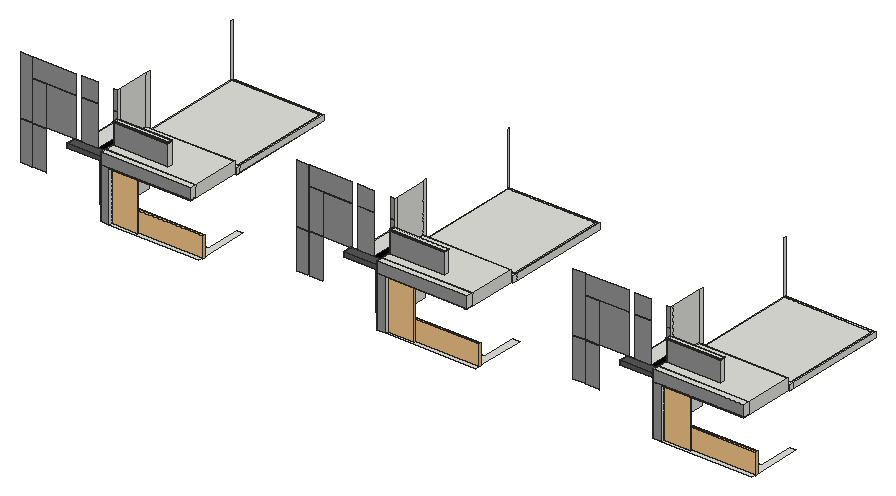
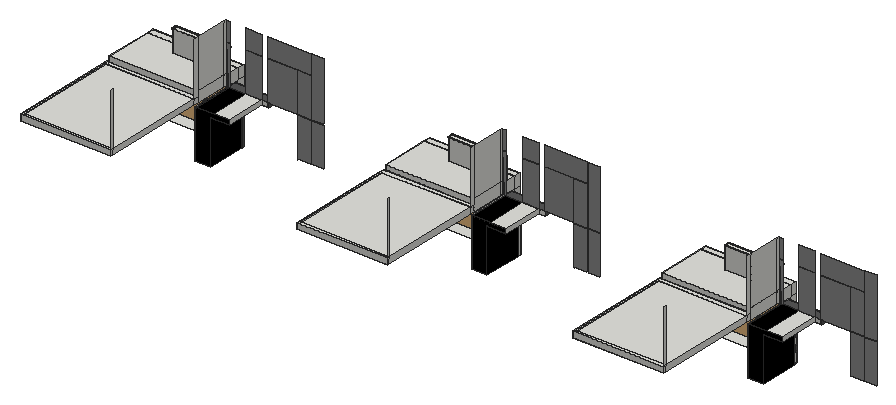
# SketchUp Ruby script. Lengths in inches.
U = 1.inch
M = Sketchup.active_model
def pt(a) = Geom::Point3d.new(a.map { |v| v * U })
def face(e, loops, mat)
  f = e.add_face(loops[0].map { |a| pt(a) })
  loops[1..].each { |l| e.add_face(l.map { |a| pt(a) }).erase! }
  f.material = f.back_material = mat if mat
  f
end
# faces: each face lists its corners as indices into pts; further lists are holes
def faces(e, pts, list, mat = nil) = list.each { |f| face(e, (f[0].is_a?(Array) ? f : [f]).map { |l| l.map { |i| pts[i] } }, mat) }
# xy, xz, yz: faces in a plane at the given z, y or x. An outline is a flat list of corners, or four numbers for a rectangle; further outlines are holes
def ring(l) = l.size == 4 ? [[l[0], l[1]], [l[2], l[1]], [l[2], l[3]], [l[0], l[3]]] : l.each_slice(2).to_a
def flat(e, list, mat, &to3) = list.each { |f| face(e, (f[0].is_a?(Array) ? f : [f]).map { |l| ring(l).map { |u, v| to3.(u, v) } }, mat) }
def xy(e, z, list, mat = nil) = flat(e, list, mat) { |x, y| [x, y, z] }
def xz(e, y, list, mat = nil) = flat(e, list, mat) { |x, z| [x, y, z] }
def yz(e, x, list, mat = nil) = flat(e, list, mat) { |y, z| [x, y, z] }
def lines(e, pts, list) = list.each { |a, b| e.add_line(pt(pts[a]), pt(pts[b])) }
# prism: a flat outline (further loops are holes) pulled along v
def prism(e, loops, v, mat = nil)
  f = face(e, loops, mat); d = Geom::Vector3d.new(v.map { |x| x * U })
  f.pushpull(f.normal.samedirection?(d) ? d.length : -d.length)
end
def box(e, o, s, mat = nil) = prism(e, [[o, [o[0] + s[0], o[1], o[2]], [o[0] + s[0], o[1] + s[1], o[2]], [o[0], o[1] + s[1], o[2]]]], [0, 0, s[2]], mat)
def at(x, y, z, deg = 0) = Geom::Transformation.translation(pt([x, y, z])) * Geom::Transformation.rotation(ORIGIN, Z_AXIS, deg.degrees)
def axes(o, x, y, z) = Geom::Transformation.new([*x, 0, *y, 0, *z, 0, *pt(o).to_a, 1])
def part(name) = M.definitions.add(name)
# library, detail: a bought-in or finely detailed component or shape, given as its bounding box
def library(name, o, s) = part(name).tap { |d| box(d.entities, o, s) }
def detail(e, o, s) = box(e.add_group.entities, o, s)
def put(e, d, t, mat = nil) = e.add_instance(d, t).tap { |i| i.material = mat if mat }
def group(e, t, mat = nil) = e.add_group.tap { |g| g.transformation = t; g.material = mat if mat }.entities
root = M.entities
M.materials.add("Glass_Tinted_Gray").color = [0, 0, 0]
M.materials["Glass_Tinted_Gray"].alpha = 0.125
M.materials.add("[0135_DarkGray]").color = [81, 81, 81]
M.materials.add("[Color C08]").color = [58, 29, 0]
M.materials.add("[Color M04]").color = [142, 142, 142]
M.materials.add("[Color M06]1").color = [86, 86, 86]
M.materials.add("[Color M07]").color = [58, 58, 58]
M.materials.add("[Color M09]").color = [0, 0, 0]
M.materials.add("[Mirror 02]").color = [229, 229, 229]
M.materials.add("[Terrazzo Light Blue]").color = [196, 214, 227]
c1 = library("Glass Railing",[0,0,0],[139.5,4.76,42])
c2 = library("Group\#2",[0,0,0],[40.6875,0.85,78])
c3 = part("PENTEK_RP Fineline 50S_Sliding_DoorCase_E1")
box(c3.entities,[0,0,0],[1.51,3.66,99.27],"[0135_DarkGray]")
c4 = part("PENTEK_RP Fineline 50S_SlidingDooe_Case_E2")
box(c4.entities,[0,0,0],[96.25,3.66,1.51],"[0135_DarkGray]")
c5 = part("pentek_RP Fineline 50S_SlidingDoor_Case")
put(c5.entities,c3,at(97.76,0,0))
put(c5.entities,c4,at(1.51,0,0))
put(c5.entities,c3,at(0,0,0))
put(c5.entities,c4,at(1.51,0,97.76))
c6 = part("PENTEK_RP Fineline 50S_SlidingDoor_GlazingBead_2")
box(c6.entities,[0,0,0],[0.56,0.59,94.39],"[0135_DarkGray]")
c7 = part("PENTEK_RP Fineline 50S_SlidingDoor_Glass")
box(c7.entities,[0,0,0],[46.58,0.16,94.39],"Glass_Tinted_Gray")
c8 = part("PENTEK_RP Fineline 50S_SlidingDoor_GlazingBead")
box(c8.entities,[0,0,0],[45.47,0.59,0.56],"[0135_DarkGray]")
c9 = part("PENTEK_RP Fineline 50S_SlidingDoor_Leaf_E1")
xy(c9.entities,0,[[0,0,0.93,1.97],[0.93,1.57,1.49,1.97]],"[0135_DarkGray]")
xy(c9.entities,96.25,[[0,0,0.93,0,0.93,1.57,1.49,1.57,1.49,1.97,0,1.97]],"[0135_DarkGray]")
xz(c9.entities,0,[[0,0,0.93,96.25]],"[0135_DarkGray]")
xz(c9.entities,1.57,[[0.93,0,1.49,95.32],[0.93,95.32,1.49,96.25]],"[0135_DarkGray]")
xz(c9.entities,1.97,[[0,0,1.49,96.25]],"[0135_DarkGray]")
yz(c9.entities,0,[[0,0,1.97,96.25]],"[0135_DarkGray]")
yz(c9.entities,0.93,[[0,0,1.57,0.93],[0,0.93,1.57,95.32],[0,95.32,1.57,96.25]],"[0135_DarkGray]")
yz(c9.entities,1.49,[[1.57,0,1.97,95.32],[1.57,95.32,1.97,96.25]],"[0135_DarkGray]")
c10 = part("PENTEK_RP Fineline 50S_SlidingDoor_Leaf_E2")
xy(c10.entities,0,[[0,0,0,1.57,0.56,1.57,0.56,1.97,46.02,1.97,46.02,1.57,46.58,1.57,46.58,0]],"[0135_DarkGray]")
xy(c10.entities,0.93,[[0,0,46.58,1.57]],"[0135_DarkGray]")
xy(c10.entities,1.49,[[0.56,1.57,46.02,1.97]],"[0135_DarkGray]")
xz(c10.entities,0,[[0,0,46.58,0.93]],"[0135_DarkGray]")
xz(c10.entities,1.57,[[0,0,0.56,0.93],[46.02,0,46.58,0.93],[0.56,0.93,46.02,1.49]],"[0135_DarkGray]")
xz(c10.entities,1.97,[[0.56,0,46.02,1.49]],"[0135_DarkGray]")
yz(c10.entities,0,[[0,0,1.57,0.93]],"[0135_DarkGray]")
yz(c10.entities,0.56,[[1.57,0,1.97,0.93],[1.57,0.93,1.97,1.49]],"[0135_DarkGray]")
yz(c10.entities,46.02,[[1.57,0,1.97,0.93],[1.57,0.93,1.97,1.49]],"[0135_DarkGray]")
yz(c10.entities,46.58,[[0,0,1.57,0.93]],"[0135_DarkGray]")
c11 = part("PENTEK_RP Fineline S_SlidingDoor_Leaf1")
put(c11.entities,c6,at(0.93,0,0.93))
put(c11.entities,c6,at(46.96,0,0.93))
put(c11.entities,c7,at(1.49,1.42,0.93))
put(c11.entities,c8,at(1.49,0,0.93))
put(c11.entities,c7,at(1.49,0.59,0.93),"[Terrazzo Light Blue]")
put(c11.entities,c9,at(0,0,0))
put(c11.entities,c9,axes([48.44,0,0],[-1,0,0],[0,1,0],[0,0,1]))
put(c11.entities,c10,axes([0.93,0,96.25],[1,0,0],[0,1,0],[0,0,-1]))
put(c11.entities,c10,at(0.93,0,0))
put(c11.entities,c8,at(1.49,0,94.77))
c12 = part("PENTEK_RP Fineline 50S_SlidingDoor_Leaf2")
put(c12.entities,c7,at(1.49,1.42,0.93))
put(c12.entities,c8,at(1.49,0,94.77))
put(c12.entities,c6,at(46.96,0,0.93))
put(c12.entities,c7,at(1.49,0.59,0.93),"[Mirror 02]")
put(c12.entities,c6,at(0.93,0,0.93))
put(c12.entities,c9,at(0,0,0))
put(c12.entities,c9,axes([48.44,0,0],[-1,0,0],[0,1,0],[0,0,1]))
put(c12.entities,c8,at(1.49,0,0.93))
put(c12.entities,c10,axes([0.93,0,96.25],[1,0,0],[0,1,0],[0,0,-1]))
put(c12.entities,c10,at(0.93,0,0))
c13 = part("PENTEK - Slimmest Steel Sliding Door / Window\#1")
put(c13.entities,c5,at(0,-1.88,-0.09))
put(c13.entities,c11,at(1.51,-2.27,1.42))
put(c13.entities,c12,at(49.32,-0.3,1.42))
xy(root,279.5625,[[281.09,243.1,299.15,256.29],[299.15,243.1,482.625,256.29],[844.22,243.1,862.27,256.29],[862.27,243.1,1045.75,256.29],[1407.34,243.1,1425.4,256.29],
  [1425.4,243.1,1608.875,256.29],[299.15,256.29,482.625,256.29,482.625,354.29,470.0625,354.29,470.0625,283.04,299.15,283.04],[862.27,256.29,1045.75,256.29,1045.75,354.29,1033.1875,354.29,1033.1875,283.04,862.27,283.04],[1425.4,256.29,1608.875,256.29,1608.875,354.29,1596.3125,354.29,1596.3125,283.04,1425.4,283.04]])
xy(root,283.9375,[[249.28,283.04,281.09,287.65],[812.4,283.04,844.22,287.65],[1375.53,283.04,1407.34,287.65]])
xy(root,283.9375,[[249.28,287.65,281.09,366.23],[812.4,287.65,844.22,366.23],[1375.53,287.65,1407.34,366.23]],"[Color M09]")
xy(root,374,[[210.82,283.04,249.28,366.23],[773.94,283.04,812.4,366.23],[1337.07,283.04,1375.53,366.23]])
xy(root,374,[[196.53,264.41,196.53,283.04,249.28,283.04,249.28,287.65,281.09,287.65,281.09,264.41],[759.65,264.41,759.65,283.04,812.4,283.04,812.4,287.65,844.22,287.65,844.22,264.41],[1322.78,264.41,1322.78,283.04,1375.53,283.04,1375.53,287.65,1407.34,287.65,1407.34,264.41]],"[Color M06]1")
xy(root,381.5,[[299.15,243.1,465.45,256.29],[862.27,243.1,1028.58,256.29],[1425.4,243.1,1591.7,256.29],[455.68,256.29,465.45,354.29],[1018.8,256.29,1028.58,354.29],
  [1581.93,256.29,1591.7,354.29]])
xy(root,382.5625,[[281.09,243.1,299.15,256.29],[299.15,243.1,465.45,256.29],[844.22,243.1,862.27,256.29],[862.27,243.1,1028.58,256.29],[1407.34,243.1,1425.4,256.29],
  [1425.4,243.1,1591.7,256.29],[281.09,256.29,299.15,256.29,299.15,354.29,285.28,354.29,285.28,283.04,281.09,283.04],[844.22,256.29,862.27,256.29,862.27,354.29,848.4,354.29,848.4,283.04,844.22,283.04],[1407.34,256.29,1425.4,256.29,1425.4,354.29,1411.53,354.29,1411.53,283.04,1407.34,283.04],[316.45,267.2,316.45,270.14,436.76,270.14,436.76,346.2,440.89,346.2,440.89,267.2],
  [879.58,267.2,879.58,270.14,999.89,270.14,999.89,346.2,1004.01,346.2,1004.01,267.2],[1442.7,267.2,1442.7,270.14,1563.01,270.14,1563.01,346.2,1567.14,346.2,1567.14,267.2],[316.85,277.89,316.85,282.58,425.1,282.58,425.1,346.77,429.22,346.77,429.22,277.89],[879.97,277.89,879.97,282.58,988.22,282.58,988.22,346.77,992.35,346.77,992.35,277.89],[1443.1,277.89,1443.1,282.58,1551.35,282.58,1551.35,346.77,1555.47,346.77,1555.47,277.89],
  [210.82,283.04,243.69,366.23],[773.94,283.04,806.82,366.23],[1337.07,283.04,1369.94,366.23],[285.28,354.29,285.28,362.98,465.45,362.98,465.45,570.3125,285.28,570.3125,285.28,574.92,470.0625,574.92,470.0625,354.29],[848.4,354.29,848.4,362.98,1028.58,362.98,1028.58,570.3125,848.4,570.3125,848.4,574.92,1033.1875,574.92,1033.1875,354.29],
  [1411.53,354.29,1411.53,362.98,1591.7,362.98,1591.7,570.3125,1411.53,570.3125,1411.53,574.92,1596.3125,574.92,1596.3125,354.29],[285.28,362.98,465.45,570.3125],[848.4,362.98,1028.58,570.3125],[1411.53,362.98,1591.7,570.3125]])
xy(root,382.5625,[[[299.15,256.29,455.68,354.29],[316.85,277.89,429.22,277.89,429.22,346.77,425.1,346.77,425.1,282.58,316.85,282.58],[316.45,267.2,440.89,267.2,440.89,346.2,436.76,346.2,436.76,270.14,316.45,270.14]],[[862.27,256.29,1018.8,354.29],[879.97,277.89,992.35,277.89,992.35,346.77,988.22,346.77,988.22,282.58,879.97,282.58],[879.58,267.2,1004.01,267.2,1004.01,346.2,999.89,346.2,999.89,270.14,879.58,270.14]],[[1425.4,256.29,1581.93,354.29],[1443.1,277.89,1555.47,277.89,1555.47,346.77,1551.35,346.77,1551.35,282.58,1443.1,282.58],[1442.7,267.2,1567.14,267.2,1567.14,346.2,1563.01,346.2,1563.01,270.14,1442.7,270.14]]],"[Color C08]")
xy(root,382.5625,[[196.53,264.41,281.09,283.04],[759.65,264.41,844.22,283.04],[1322.78,264.41,1407.34,283.04]],"[Color M06]1")
xy(root,382.5625,[[243.69,283.04,277.35,366.23],[277.35,283.04,281.09,366.23],[806.82,283.04,840.48,366.23],[840.48,283.04,844.22,366.23],[1369.94,283.04,1403.6,366.23],
  [1403.6,283.04,1407.34,366.23]],"[Color M09]")
xy(root,394.5,[[285.28,354.29,470.0625,354.29,470.0625,574.92,285.28,574.92,285.28,570.3125,465.45,570.3125,465.45,362.98,285.28,362.98],[848.4,354.29,1033.1875,354.29,1033.1875,574.92,848.4,574.92,848.4,570.3125,1028.58,570.3125,1028.58,362.98,848.4,362.98],[1411.53,354.29,1596.3125,354.29,1596.3125,574.92,1411.53,574.92,1411.53,570.3125,1591.7,570.3125,1591.7,362.98,1411.53,362.98],[285.28,362.98,465.45,570.3125],[848.4,362.98,1028.58,570.3125],
  [1411.53,362.98,1591.7,570.3125]])
xy(root,405.25,[[281.09,243.1,465.45,256.29],[844.22,243.1,1028.58,256.29],[1407.34,243.1,1591.7,256.29],[281.09,256.29,465.45,256.29,465.45,354.29,285.28,354.29,285.28,283.04,393.75,283.04,393.75,274.41,283.19,274.41,283.19,283.04,281.09,283.04],[844.22,256.29,1028.58,256.29,1028.58,354.29,848.4,354.29,848.4,283.04,956.87,283.04,956.87,274.41,846.31,274.41,846.31,283.04,844.22,283.04],
  [1407.34,256.29,1591.7,256.29,1591.7,354.29,1411.53,354.29,1411.53,283.04,1520,283.04,1520,274.41,1409.44,274.41,1409.44,283.04,1407.34,283.04]])
xy(root,448.0625,[[283.19,274.41,393.75,283.04],[846.31,274.41,956.87,283.04],[1409.44,274.41,1520,283.04]])
xy(root,448.0625,[[283.19,272.66,393.75,274.41],[393.75,272.66,395.19,274.41],[846.31,272.66,956.87,274.41],[956.87,272.66,958.31,274.41],[1409.44,272.66,1520,274.41],
  [1520,272.66,1521.44,274.41],[393.75,274.41,395.19,283.04],[956.87,274.41,958.31,283.04],[1520,274.41,1521.44,283.04]],"[Color M07]")
xy(root,449.5,[[283.19,272.66,393.75,274.41],[393.75,272.66,395.19,274.41],[846.31,272.66,956.87,274.41],[956.87,272.66,958.31,274.41],[1409.44,272.66,1520,274.41],
  [1520,272.66,1521.44,274.41],[283.19,274.41,393.75,283.04],[393.75,274.41,395.19,283.04],[846.31,274.41,956.87,283.04],[956.87,274.41,958.31,283.04],
  [1409.44,274.41,1520,283.04],[1520,274.41,1521.44,283.04]])
xz(root,243.1,[[299.15,381.5,465.45,382.5625],[862.27,381.5,1028.58,382.5625],[1425.4,381.5,1591.7,382.5625]])
xz(root,243.1,[[281.09,279.5625,299.15,382.5625],[844.22,279.5625,862.27,382.5625],[1407.34,279.5625,1425.4,382.5625],[281.09,382.5625,465.45,405.25],[844.22,382.5625,1028.58,405.25],
  [1407.34,382.5625,1591.7,405.25]],"[Color M04]")
xz(root,256.29,[[281.09,279.5625,299.15,382.5625],[844.22,279.5625,862.27,382.5625],[1407.34,279.5625,1425.4,382.5625],[299.15,381.5,455.68,382.5625],[455.68,381.5,465.45,382.5625],
  [862.27,381.5,1018.8,382.5625],[1018.8,381.5,1028.58,382.5625],[1425.4,381.5,1581.93,382.5625],[1581.93,381.5,1591.7,382.5625],[281.09,382.5625,465.45,405.25],
  [844.22,382.5625,1028.58,405.25],[1407.34,382.5625,1591.7,405.25]])
xz(root,264.41,[[196.53,374,281.09,382.5625],[759.65,374,844.22,382.5625],[1322.78,374,1407.34,382.5625]],"[Color M06]1")
xz(root,272.66,[[283.19,448.0625,393.75,449.5],[393.75,448.0625,395.19,449.5],[846.31,448.0625,956.87,449.5],[956.87,448.0625,958.31,449.5],[1409.44,448.0625,1520,449.5],
  [1520,448.0625,1521.44,449.5]],"[Color M07]")
xz(root,274.41,[[283.19,448.0625,393.75,449.5],[393.75,448.0625,395.19,449.5],[846.31,448.0625,956.87,449.5],[956.87,448.0625,958.31,449.5],[1409.44,448.0625,1520,449.5],
  [1520,448.0625,1521.44,449.5]])
xz(root,274.41,[[283.19,405.25,393.75,448.0625],[846.31,405.25,956.87,448.0625],[1409.44,405.25,1520,448.0625]],"[Color M04]")
xz(root,283.04,[[196.53,374,198.84,382.5625],[198.84,374,210.82,382.5625],[759.65,374,761.97,382.5625],[761.97,374,773.94,382.5625],[1322.78,374,1325.09,382.5625],
  [1325.09,374,1337.07,382.5625],[281.09,382.5625,285.28,382.5625,285.28,448.0625,283.19,448.0625,283.19,405.25,281.09,405.25],[844.22,382.5625,848.4,382.5625,848.4,448.0625,846.31,448.0625,846.31,405.25,844.22,405.25],[1407.34,382.5625,1411.53,382.5625,1411.53,448.0625,1409.44,448.0625,1409.44,405.25,1407.34,405.25],[285.28,405.25,393.75,448.0625],
  [848.4,405.25,956.87,448.0625],[1411.53,405.25,1520,448.0625],[283.19,448.0625,285.28,449.5],[285.28,448.0625,393.75,449.5],[393.75,448.0625,395.19,449.5],
  [846.31,448.0625,848.4,449.5],[848.4,448.0625,956.87,449.5],[956.87,448.0625,958.31,449.5],[1409.44,448.0625,1411.53,449.5],[1411.53,448.0625,1520,449.5],
  [1520,448.0625,1521.44,449.5]])
xz(root,283.04,[[86.0625,301.46,109.54,380.6],[111.72,301.46,138.73,380.6],[649.1875,301.46,672.66,380.6],[674.85,301.46,701.85,380.6],[1212.3125,301.46,1235.79,380.6],
  [1237.97,301.46,1264.98,380.6],[86.0625,382.5625,109.54,502.5625],[111.72,382.5625,138.73,462.57],[140.54,382.5625,198.84,462.57],[210.82,382.5625,243.69,462.57],
  [277.35,382.5625,281.09,382.5625,281.09,405.25,283.19,405.25,283.19,449.5,285.28,449.5,285.28,462.57,277.35,462.57],[649.1875,382.5625,672.66,502.5625],[674.85,382.5625,701.85,462.57],[703.67,382.5625,761.97,462.57],[773.94,382.5625,806.82,462.57],
  [840.48,382.5625,844.22,382.5625,844.22,405.25,846.31,405.25,846.31,449.5,848.4,449.5,848.4,462.57,840.48,462.57],[1212.3125,382.5625,1235.79,502.5625],[1237.97,382.5625,1264.98,462.57],[1266.79,382.5625,1325.09,462.57],[1337.07,382.5625,1369.94,462.57],
  [1403.6,382.5625,1407.34,382.5625,1407.34,405.25,1409.44,405.25,1409.44,449.5,1411.53,449.5,1411.53,462.57,1403.6,462.57],[111.72,463.9375,198.84,502.5625],[210.82,463.9375,243.69,502.5625],[277.35,463.9375,285.28,502.5625],[674.85,463.9375,761.97,502.5625],
  [773.94,463.9375,806.82,502.5625],[840.48,463.9375,848.4,502.5625],[1237.97,463.9375,1325.09,502.5625],[1337.07,463.9375,1369.94,502.5625],[1403.6,463.9375,1411.53,502.5625]],"[Color M04]")
xz(root,287.65,[[280.83,283.9375,281.09,374],[843.96,283.9375,844.22,374],[1407.08,283.9375,1407.34,374]])
xz(root,354.29,[[455.68,381.5,465.45,382.5625],[1018.8,381.5,1028.58,382.5625],[1581.93,381.5,1591.7,382.5625],[285.28,382.5625,465.45,394.5],[465.45,382.5625,470.0625,394.5],
  [848.4,382.5625,1028.58,394.5],[1028.58,382.5625,1033.1875,394.5],[1411.53,382.5625,1591.7,394.5],[1591.7,382.5625,1596.3125,394.5],[285.28,394.5,465.45,405.25],
  [848.4,394.5,1028.58,405.25],[1411.53,394.5,1591.7,405.25]])
xz(root,362.98,[[285.28,382.5625,465.45,394.5],[848.4,382.5625,1028.58,394.5],[1411.53,382.5625,1591.7,394.5]])
xz(root,366.23,[[249.28,283.9375,281.09,283.9375,281.09,382.5625,210.82,382.5625,210.82,374,249.28,374],[812.4,283.9375,844.22,283.9375,844.22,382.5625,773.94,382.5625,773.94,374,812.4,374],[1375.53,283.9375,1407.34,283.9375,1407.34,382.5625,1337.07,382.5625,1337.07,374,1375.53,374]],"[Color M09]")
xz(root,574.92,[[285.28,382.5625,470.0625,394.5],[848.4,382.5625,1033.1875,394.5],[1411.53,382.5625,1596.3125,394.5]])
yz(root,196.53,[[264.41,374,283.04,382.5625]],"[Color M06]1")
yz(root,210.82,[[283.04,374,366.23,382.5625]])
yz(root,249.28,[[283.04,283.9375,287.65,374]])
yz(root,249.28,[[287.65,283.9375,366.23,374]],"[Color M09]")
yz(root,281.09,[[243.1,279.5625,256.29,382.5625],[283.04,283.9375,287.65,374],[287.65,283.9375,366.23,374],[264.41,374,283.04,382.5625],[283.04,374,366.23,382.5625],
  [243.1,382.5625,256.29,405.25],[256.29,382.5625,283.04,405.25]])
yz(root,283.19,[[274.41,405.25,283.04,448.0625],[272.66,448.0625,274.41,449.5],[274.41,448.0625,283.04,449.5]])
yz(root,285.28,[[283.04,382.5625,287.65,405.25],[287.65,382.5625,354.29,405.25],[354.29,382.5625,362.98,394.5],[362.98,382.5625,570.3125,394.5],[570.3125,382.5625,574.92,394.5],
  [354.29,394.5,362.98,502.5625],[570.3125,394.5,574.92,502.5625],[283.04,405.25,287.65,502.5625],[287.65,405.25,354.29,502.5625]])
yz(root,299.15,[[243.1,279.5625,256.29,381.5],[243.1,381.5,256.29,382.5625]])
yz(root,393.75,[[274.41,405.25,283.04,448.0625],[272.66,448.0625,274.41,449.5],[274.41,448.0625,283.04,449.5]])
yz(root,395.19,[[272.66,448.0625,274.41,449.5],[274.41,448.0625,283.04,449.5]],"[Color M07]")
yz(root,455.68,[[256.29,381.5,354.29,382.5625]])
yz(root,465.45,[[243.1,381.5,256.29,382.5625],[256.29,381.5,354.29,405.25],[243.1,382.5625,256.29,405.25],[362.98,382.5625,570.3125,394.5]])
yz(root,470.0625,[[354.29,382.5625,362.98,394.5],[362.98,382.5625,574.92,394.5]])
yz(root,759.65,[[264.41,374,283.04,382.5625]],"[Color M06]1")
yz(root,773.94,[[283.04,374,366.23,382.5625]])
yz(root,812.4,[[283.04,283.9375,287.65,374]])
yz(root,812.4,[[287.65,283.9375,366.23,374]],"[Color M09]")
yz(root,844.22,[[243.1,279.5625,256.29,382.5625],[283.04,283.9375,287.65,374],[287.65,283.9375,366.23,374],[264.41,374,283.04,382.5625],[283.04,374,366.23,382.5625],
  [243.1,382.5625,256.29,405.25],[256.29,382.5625,283.04,405.25]])
yz(root,846.31,[[274.41,405.25,283.04,448.0625],[272.66,448.0625,274.41,449.5],[274.41,448.0625,283.04,449.5]])
yz(root,848.4,[[283.04,382.5625,287.65,405.25],[287.65,382.5625,354.29,405.25],[354.29,382.5625,362.98,394.5],[362.98,382.5625,570.3125,394.5],[570.3125,382.5625,574.92,394.5],
  [354.29,394.5,362.98,502.5625],[570.3125,394.5,574.92,502.5625],[283.04,405.25,287.65,502.5625],[287.65,405.25,354.29,502.5625]])
yz(root,862.27,[[243.1,279.5625,256.29,381.5],[243.1,381.5,256.29,382.5625]])
yz(root,956.87,[[274.41,405.25,283.04,448.0625],[272.66,448.0625,274.41,449.5],[274.41,448.0625,283.04,449.5]])
yz(root,958.31,[[272.66,448.0625,274.41,449.5],[274.41,448.0625,283.04,449.5]],"[Color M07]")
yz(root,1018.8,[[256.29,381.5,354.29,382.5625]])
yz(root,1028.58,[[243.1,381.5,256.29,382.5625],[256.29,381.5,354.29,405.25],[243.1,382.5625,256.29,405.25],[362.98,382.5625,570.3125,394.5]])
yz(root,1033.1875,[[354.29,382.5625,362.98,394.5],[362.98,382.5625,574.92,394.5]])
yz(root,1322.78,[[264.41,374,283.04,382.5625]],"[Color M06]1")
yz(root,1337.07,[[283.04,374,366.23,382.5625]])
yz(root,1375.53,[[283.04,283.9375,287.65,374]])
yz(root,1375.53,[[287.65,283.9375,366.23,374]],"[Color M09]")
yz(root,1407.34,[[243.1,279.5625,256.29,382.5625],[283.04,283.9375,287.65,374],[287.65,283.9375,366.23,374],[264.41,374,283.04,382.5625],[283.04,374,366.23,382.5625],
  [243.1,382.5625,256.29,405.25],[256.29,382.5625,283.04,405.25]])
yz(root,1409.44,[[274.41,405.25,283.04,448.0625],[272.66,448.0625,274.41,449.5],[274.41,448.0625,283.04,449.5]])
yz(root,1411.53,[[283.04,382.5625,287.65,405.25],[287.65,382.5625,354.29,405.25],[354.29,382.5625,362.98,394.5],[362.98,382.5625,570.3125,394.5],[570.3125,382.5625,574.92,394.5],
  [354.29,394.5,362.98,502.5625],[570.3125,394.5,574.92,502.5625],[283.04,405.25,287.65,502.5625],[287.65,405.25,354.29,502.5625]])
yz(root,1425.4,[[243.1,279.5625,256.29,381.5],[243.1,381.5,256.29,382.5625]])
yz(root,1520,[[274.41,405.25,283.04,448.0625],[272.66,448.0625,274.41,449.5],[274.41,448.0625,283.04,449.5]])
yz(root,1521.44,[[272.66,448.0625,274.41,449.5],[274.41,448.0625,283.04,449.5]],"[Color M07]")
yz(root,1581.93,[[256.29,381.5,354.29,382.5625]])
yz(root,1591.7,[[243.1,381.5,256.29,382.5625],[256.29,381.5,354.29,405.25],[243.1,382.5625,256.29,405.25],[362.98,382.5625,570.3125,394.5]])
yz(root,1596.3125,[[354.29,382.5625,362.98,394.5],[362.98,382.5625,574.92,394.5]])
p = [[701.875,283.04,301.46],[701.85,283.04,301.46],[701.85,283.04,299.14],[701.875,283.04,299.14],[1265,283.04,301.46],[1264.98,283.04,301.46],
  [1264.98,283.04,299.14],[1265,283.04,299.14],[138.73,283.04,299.14],[138.75,283.04,299.14],[138.75,283.04,301.46],[138.73,283.04,301.46]]
lines(root,p,[[0,1],[2,3],[4,5],[6,7],[8,9],[10,11]])
put(root,c1,axes([862.27,252.1,277.89],[1.31526,0,0],[0,1,0],[0,0,1]))
put(root,c1,axes([299.15,252.1,277.89],[1.31526,0,0],[0,1,0],[0,0,1]))
put(root,c1,axes([1425.4,252.1,277.89],[1.31526,0,0],[0,1,0],[0,0,1]))
put(root,c2,axes([862.27,248.58,279.6],[1.32,0,0],[0,1.32,0],[0,0,1.32]))
put(root,c2,axes([299.15,248.58,279.6],[1.32,0,0],[0,1.32,0],[0,0,1.32]))
put(root,c2,axes([1425.4,248.58,279.6],[1.32,0,0],[0,1.32,0],[0,0,1.32]))
put(root,c13,axes([812.4,283.04,283.93],[0.32046,0,0],[0,1,0],[0,0,0.90815]))
put(root,c13,axes([249.28,283.04,283.93],[0.32046,0,0],[0,1,0],[0,0,0.90815]))
put(root,c13,axes([1375.53,283.04,283.93],[0.32046,0,0],[0,1,0],[0,0,0.90815]))
